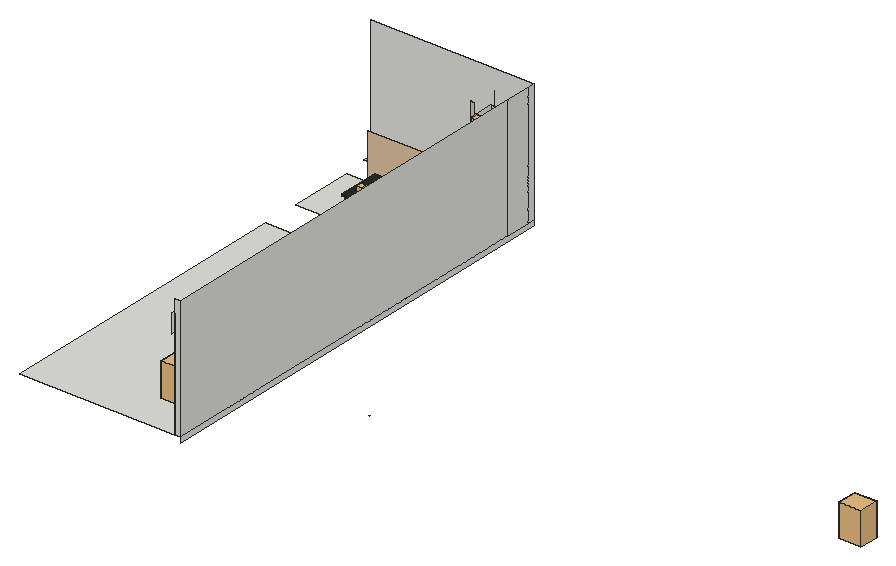
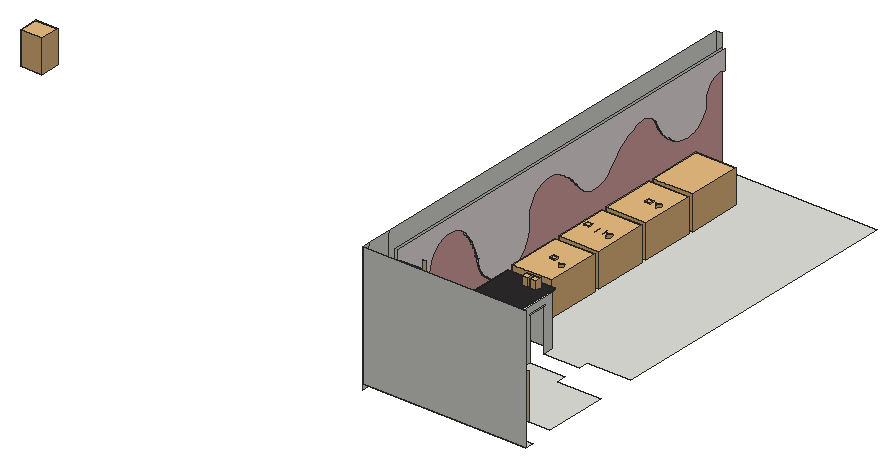
# SketchUp Ruby script. Lengths in inches.
U = 1.inch
M = Sketchup.active_model
def pt(a) = Geom::Point3d.new(a.map { |v| v * U })
def face(e, loops, mat)
  f = e.add_face(loops[0].map { |a| pt(a) })
  loops[1..].each { |l| e.add_face(l.map { |a| pt(a) }).erase! }
  f.material = f.back_material = mat if mat
  f
end
# faces: each face lists its corners as indices into pts; further lists are holes
def faces(e, pts, list, mat = nil) = list.each { |f| face(e, (f[0].is_a?(Array) ? f : [f]).map { |l| l.map { |i| pts[i] } }, mat) }
# xy, xz, yz: faces in a plane at the given z, y or x. An outline is a flat list of corners, or four numbers for a rectangle; further outlines are holes
def ring(l) = l.size == 4 ? [[l[0], l[1]], [l[2], l[1]], [l[2], l[3]], [l[0], l[3]]] : l.each_slice(2).to_a
def flat(e, list, mat, &to3) = list.each { |f| face(e, (f[0].is_a?(Array) ? f : [f]).map { |l| ring(l).map { |u, v| to3.(u, v) } }, mat) }
def xy(e, z, list, mat = nil) = flat(e, list, mat) { |x, y| [x, y, z] }
def xz(e, y, list, mat = nil) = flat(e, list, mat) { |x, z| [x, y, z] }
def yz(e, x, list, mat = nil) = flat(e, list, mat) { |y, z| [x, y, z] }
def lines(e, pts, list) = list.each { |a, b| e.add_line(pt(pts[a]), pt(pts[b])) }
# prism: a flat outline (further loops are holes) pulled along v
def prism(e, loops, v, mat = nil)
  f = face(e, loops, mat); d = Geom::Vector3d.new(v.map { |x| x * U })
  f.pushpull(f.normal.samedirection?(d) ? d.length : -d.length)
end
def box(e, o, s, mat = nil) = prism(e, [[o, [o[0] + s[0], o[1], o[2]], [o[0] + s[0], o[1] + s[1], o[2]], [o[0], o[1] + s[1], o[2]]]], [0, 0, s[2]], mat)
def at(x, y, z, deg = 0) = Geom::Transformation.translation(pt([x, y, z])) * Geom::Transformation.rotation(ORIGIN, Z_AXIS, deg.degrees)
def axes(o, x, y, z) = Geom::Transformation.new([*x, 0, *y, 0, *z, 0, *pt(o).to_a, 1])
def part(name) = M.definitions.add(name)
# library, detail: a bought-in or finely detailed component or shape, given as its bounding box
def library(name, o, s) = part(name).tap { |d| box(d.entities, o, s) }
def detail(e, o, s) = box(e.add_group.entities, o, s)
def put(e, d, t, mat = nil) = e.add_instance(d, t).tap { |i| i.material = mat if mat }
def group(e, t, mat = nil) = e.add_group.tap { |g| g.transformation = t; g.material = mat if mat }.entities
root = M.entities
M.materials.add("Generic").color = [224, 169, 169]
M.materials.add("Generic\#1").color = [44, 42, 42]
M.materials.add("Generic\#2").color = [246, 234, 234]
M.materials.add("Generic\#3").color = [224, 196, 161]
M.materials.add("Material__1").color = [51, 42, 44]
M.materials.add("Material__2").color = [97, 132, 37]
M.materials.add("[Color M00]").color = [255, 255, 255]
M.materials.add("[Mirror 02]").color = [230, 230, 230]
M.materials.add("[Translucent Glass Tinted]").color = [7, 201, 240]
M.materials["[Translucent Glass Tinted]"].alpha = 0.48
c1 = library("coffee+cup+lid",[0,0,0.03],[3.7,3.7,4.95])
c2 = library("\#1",[-138.85,-135.75,0],[277.7,270.97,9.64])
c3 = library("\#2",[-34.84,-73.35,-33.91],[69.68,146.26,68.31])
c4 = library("\#5",[-4127.85,-1300.75,-2324.72],[5349.84,4521.24,5423.31])
c5 = part("\#3")
put(c5.entities,c4,at(450.18,-1111.4375,0),"Material__2")
c6 = part("12")
put(c6.entities,c2,axes([-49.79,-36.9375,349.64],[0.59279,0,0],[0,0.59279,0],[0,0,0.59279]),"Material__1")
put(c6.entities,c3,axes([-39.24,-18.18,177.19],[1.20819,-2.09264,0],[0,0,2.41638],[2.09264,1.20819,0]))
put(c6.entities,c5,axes([-83.44,-46.04,442.44],[-0.03636,-0.03293,-0.01473],[-0.00083,-0.02391,0.05549],[0.02997,-0.02791,-0.01158]))
c7 = part("Group\#585")
xy(c7.entities,2.68,[[0,0,4.06,4.25]],"[Color M00]")
xz(c7.entities,0,[[0,0,4.06,2.68]],"[Color M00]")
xz(c7.entities,4.25,[[0,0,4.06,2.68]],"[Color M00]")
yz(c7.entities,0,[[0,0,4.25,2.68]],"[Color M00]")
yz(c7.entities,4.06,[[0,0,4.25,2.68]],"[Color M00]")
c8 = library("Tissue box",[0,0,0],[4.59,4,6.84])
c9 = library("Group\#665",[0,0,0],[25.17,25.17,22.5])
c10 = library("Group\#77",[0,0,0],[37.5,57.43,36.06])
c11 = library("Group\#78",[0,0,0],[37.5,57.43,36.06])
c12 = library("Group\#79",[0,0,0],[37.5,57.43,36.06])
c13 = library("Group\#80",[0,0,0],[37.5,57.43,36.06])
c14 = library("Group\#661",[0,0,0],[62.4,40.28,25.88])
xy(root,0,[[184.0625,0,190,453.375],[180.77,453.375,190,481.125],[153.2,476.9375,180.77,476.9375,180.77,481.125,190,481.125,190,490.125,9,490.125,9,481.125,153.2,481.125]])
xy(root,58.4375,[[97.8125,338.55,149.9375,340.55],[97.8125,340.55,99.75,382.3],[99.75,340.55,147.9375,382.3],[147.9375,340.55,149.9375,384.3],[97.8125,382.3,147.9375,384.3]])
xy(root,60.3125,[[97.8125,338.55,149.9375,384.3]],"Generic\#1")
xz(root,0,[[184.0625,0,190,135.25]])
xz(root,338.55,[[97.8125,58.4375,149.9375,60.3125]],"Generic\#1")
xz(root,340.55,[[99.75,0,147.9375,58.4375]])
xz(root,382.3,[[99.75,0,147.9375,58.4375]])
xz(root,384.3,[[97.8125,58.4375,149.9375,60.3125]])
xz(root,453.375,[[180.77,0,184.0625,0,184.0625,75.96,180.9375,75.96,180.9375,120,180.77,120],[184.0625,0,190,67.8125]])
xz(root,453.375,[[34.875,0,153.2,0,153.2,120,149.93,120,149.93,89.18,150.375,89.18,150.375,71.49,150.42,68.36,150.42,50.68,35.21,50.68,35.29,46.12]],"Generic\#3")
xz(root,476.9375,[[153.2,0,180.77,107.14]])
xz(root,490.125,[[9,0,190,135.25]])
yz(root,99.75,[[340.55,0,340.55,58.4375,382.3,58.4375,382.3,0,371.55,0,371.55,47.6875,372.8,47.6875,372.8,48.3125,350.05,48.3125,350.05,47.6875,351.3,47.6875,351.3,0],[350.05,47.6875,372.8,48.3125]])
yz(root,147.9375,[[340.55,0,382.3,58.4375]])
yz(root,149.9375,[[338.55,58.4375,384.3,60.3125]],"Generic\#1")
yz(root,150.42,[[453.375,50.68,476.6875,68.36]],"Generic\#3")
yz(root,150.79,[[453.375,45.99,467.1875,46.12]])
yz(root,153.2,[[453.375,0,476.9375,107.14]])
yz(root,180.77,[[453.375,0,476.9375,107.14]])
yz(root,180.9375,[[309.3,28.65,300.48,28.89,292.02,31.36,284.45,35.875,278.27,42.16,273.87,49.8,271.54,58.3,271.43,67.11,271.55,72.61,270.64,78.03,268.73,83.18,265.88,87.89,262.21,91.98,257.84,95.3125,252.92,97.77,247.63,99.26,242.16,99.73,236.6875,99.18,231.42,97.61,226.54,95.08,224.11,93.46,221.73,91.77,219.41,90.01,217.14,88.18,214.93,86.28,212.78,84.31,210.68,82.27,208.66,80.17,206.7,78.01,204.8,75.8,202.98,73.52,201.22,71.1875,198.44,67.94,195.19,65.17,191.55,62.95,187.6,61.31,183.45,60.32,179.1875,59.98,174.93,60.32,170.78,61.31,166.83,62.95,163.1875,65.17,159.9375,67.94,157.16,71.1875,154.72,74.36,152.1,77.39,149.34,80.28,146.41,83.01,143.35,85.58,140.15,87.99,136.83,90.22,133.39,92.26,129.85,94.12,126.21,95.79,122.48,97.25,118.6875,98.51,116.17,99.11,113.59,99.4,111,99.36,108.43,99.01,105.93,98.35,103.52,97.38,101.25,96.13,99.15,94.61,97.26,92.84,95.59,90.85,94.18,88.68,93.05,86.35,91.38,82.68,89.4375,79.15,87.23,75.77,84.78,72.57,82.09,69.57,79.1875,66.78,76.08,64.21,72.79,61.88,69.33,59.8125,65.72,58.01,61.99,56.48,58.16,55.24,54.1875,54.44,50.14,54.28,46.12,54.74,42.22,55.83,38.53,57.51,35.16,59.75,32.17,62.48,29.64,65.65,27.64,69.17,26.21,72.96,25.39,76.92,25.2,80.97,25.04,84,24.39,86.97,23.27,89.8,21.69,92.4,19.72,94.71,17.39,96.67,14.78,98.22,11.95,99.33,8.97,99.96,5.9375,100.09,2.92,99.73,0,98.88,0,120,453.375,120,453.375,75.96,452.625,70.25,450.42,64.92,446.91,60.36,442.34,56.85,437.02,54.65,431.3125,53.89,425.6,54.65,420.28,56.85,415.71,60.36,412.21,64.92,410,70.25,409.25,75.96,408.67,81.6875,406.96,87.1875,404.1875,92.23,400.46,96.625,395.93,100.18,390.79,102.77,385.23,104.27,379.48,104.64,373.77,103.84,368.34,101.93,363.4,98.97,359.15,95.08,356.78,92.31,354.54,89.43,352.42,86.46,350.45,83.4,348.6,80.25,346.9,77.02,345.35,73.73,343.94,70.36,342.6875,66.9375,341.58,63.46,340.64,59.9375,339.85,56.38,337.04,48.02,332.22,40.64,325.7,34.72,317.89,30.63]],"Generic\#2")
yz(root,184.0625,[[309.3,28.65,317.89,30.63,325.7,34.72,332.22,40.64,337.04,48.02,339.85,56.38,340.64,59.9375,341.58,63.46,342.6875,66.9375,343.94,70.36,345.35,73.73,346.9,77.02,348.6,80.25,350.45,83.4,352.42,86.46,354.54,89.43,356.78,92.31,359.15,95.08,363.4,98.97,368.34,101.93,373.77,103.84,379.48,104.64,385.23,104.27,390.79,102.77,395.93,100.18,400.46,96.625,404.1875,92.23,406.96,87.1875,408.67,81.6875,409.25,75.96,410,70.25,412.21,64.92,415.71,60.36,420.28,56.85,425.6,54.65,431.3125,53.89,437.02,54.65,442.34,56.85,446.91,60.36,450.42,64.92,452.625,70.25,453.375,75.96,453.375,120,0,120,0,98.88,2.92,99.73,5.9375,100.09,8.97,99.96,11.95,99.33,14.78,98.22,17.39,96.67,19.72,94.71,21.69,92.4,23.27,89.8,24.39,86.97,25.04,84,25.2,80.97,25.39,76.92,26.21,72.96,27.64,69.17,29.64,65.65,32.17,62.48,35.16,59.75,38.53,57.51,42.22,55.83,46.12,54.74,50.14,54.28,54.1875,54.44,58.16,55.24,61.99,56.48,65.72,58.01,69.33,59.8125,72.79,61.88,76.08,64.21,79.1875,66.78,82.09,69.57,84.78,72.57,87.23,75.77,89.4375,79.15,91.38,82.68,93.05,86.35,94.18,88.68,95.59,90.85,97.26,92.84,99.15,94.61,101.25,96.13,103.52,97.38,105.93,98.35,108.43,99.01,111,99.36,113.59,99.4,116.17,99.11,118.6875,98.51,122.48,97.25,126.21,95.79,129.85,94.12,133.39,92.26,136.83,90.22,140.15,87.99,143.35,85.58,146.41,83.01,149.34,80.28,152.1,77.39,154.72,74.36,157.16,71.1875,159.9375,67.94,163.1875,65.17,166.83,62.95,170.78,61.31,174.93,60.32,179.1875,59.98,183.45,60.32,187.6,61.31,191.55,62.95,195.19,65.17,198.44,67.94,201.22,71.1875,202.98,73.52,204.8,75.8,206.7,78.01,208.66,80.17,210.68,82.27,212.78,84.31,214.93,86.28,217.14,88.18,219.41,90.01,221.73,91.77,224.11,93.46,226.54,95.08,231.42,97.61,236.6875,99.18,242.16,99.73,247.63,99.26,252.92,97.77,257.84,95.3125,262.21,91.98,265.88,87.89,268.73,83.18,270.64,78.03,271.55,72.61,271.43,67.11,271.54,58.3,273.87,49.8,278.27,42.16,284.45,35.875,292.02,31.36,300.48,28.89]])
yz(root,184.0625,[[0,0,0,98.88,2.92,99.73,5.9375,100.09,8.97,99.96,11.95,99.33,14.78,98.22,17.39,96.67,19.72,94.71,21.69,92.4,23.27,89.8,24.39,86.97,25.04,84,25.2,80.97,25.39,76.92,26.21,72.96,27.64,69.17,29.64,65.65,32.17,62.48,35.16,59.75,38.53,57.51,42.22,55.83,46.12,54.74,50.14,54.28,54.1875,54.44,58.16,55.24,61.99,56.48,65.72,58.01,69.33,59.8125,72.79,61.88,76.08,64.21,79.1875,66.78,82.09,69.57,84.78,72.57,87.23,75.77,89.4375,79.15,91.38,82.68,93.05,86.35,94.18,88.68,95.59,90.85,97.26,92.84,99.15,94.61,101.25,96.13,103.52,97.38,105.93,98.35,108.43,99.01,111,99.36,113.59,99.4,116.17,99.11,118.6875,98.51,122.48,97.25,126.21,95.79,129.85,94.12,133.39,92.26,136.83,90.22,140.15,87.99,143.35,85.58,146.41,83.01,149.34,80.28,152.1,77.39,154.72,74.36,157.16,71.1875,159.9375,67.94,163.1875,65.17,166.83,62.95,170.78,61.31,174.93,60.32,179.1875,59.98,183.45,60.32,187.6,61.31,191.55,62.95,195.19,65.17,198.44,67.94,201.22,71.1875,202.98,73.52,204.8,75.8,206.7,78.01,208.66,80.17,210.68,82.27,212.78,84.31,214.93,86.28,217.14,88.18,219.41,90.01,221.73,91.77,224.11,93.46,226.54,95.08,231.42,97.61,236.6875,99.18,242.16,99.73,247.63,99.26,252.92,97.77,257.84,95.3125,262.21,91.98,265.88,87.89,268.73,83.18,270.64,78.03,271.55,72.61,271.43,67.11,271.54,58.3,273.87,49.8,278.27,42.16,284.45,35.875,292.02,31.36,300.48,28.89,309.3,28.65,317.89,30.63,325.7,34.72,332.22,40.64,337.04,48.02,339.85,56.38,340.64,59.9375,341.58,63.46,342.6875,66.9375,343.94,70.36,345.35,73.73,346.9,77.02,348.6,80.25,350.45,83.4,352.42,86.46,354.54,89.43,356.78,92.31,359.15,95.08,363.4,98.97,368.34,101.93,373.77,103.84,379.48,104.64,385.23,104.27,390.79,102.77,395.93,100.18,400.46,96.625,404.1875,92.23,406.96,87.1875,408.67,81.6875,409.25,75.96,410,70.25,412.21,64.92,415.71,60.36,420.28,56.85,425.6,54.65,431.3125,53.89,437.02,54.65,442.34,56.85,446.91,60.36,450.42,64.92,452.625,70.25,453.375,75.96,453.375,0]],"Generic")
yz(root,190,[[0,-6,490.125,0],[0,0,453.375,135.25],[453.375,0,481.125,135.25],[481.125,0,490.125,135.25]])
p = [[184.0625,309.3,28.65],[184.0625,300.48,28.89],[180.9375,300.48,28.89],[180.9375,309.3,28.65],[184.0625,317.89,30.63],[180.9375,317.89,30.63],
  [184.0625,292.02,31.36],[180.9375,292.02,31.36],[184.0625,325.7,34.72],[180.9375,325.7,34.72],[184.0625,284.45,35.875],[180.9375,284.45,35.875],
  [184.0625,332.22,40.64],[180.9375,332.22,40.64],[184.0625,278.27,42.16],[180.9375,278.27,42.16],[184.0625,337.04,48.02],[180.9375,337.04,48.02],
  [184.0625,273.87,49.8],[180.9375,273.87,49.8],[184.0625,339.85,56.38],[180.9375,339.85,56.38],[184.0625,271.54,58.3],[180.9375,271.54,58.3],
  [184.0625,431.3125,53.89],[184.0625,425.6,54.65],[180.9375,425.6,54.65],[180.9375,431.3125,53.89],[184.0625,437.02,54.65],[180.9375,437.02,54.65],
  [184.0625,50.14,54.28],[184.0625,46.12,54.74],[180.9375,46.12,54.74],[180.9375,50.14,54.28],[184.0625,54.1875,54.44],[180.9375,54.1875,54.44],
  [184.0625,58.16,55.24],[180.9375,58.16,55.24],[184.0625,420.28,56.85],[180.9375,420.28,56.85],[184.0625,442.34,56.85],[180.9375,442.34,56.85],
  [184.0625,42.22,55.83],[180.9375,42.22,55.83],[184.0625,61.99,56.48],[180.9375,61.99,56.48],[184.0625,38.53,57.51],[180.9375,38.53,57.51],
  [184.0625,340.64,59.9375],[180.9375,340.64,59.9375],[184.0625,65.72,58.01],[180.9375,65.72,58.01],[184.0625,415.71,60.36],[180.9375,415.71,60.36],
  [184.0625,446.91,60.36],[180.9375,446.91,60.36],[184.0625,35.16,59.75],[180.9375,35.16,59.75],[184.0625,69.33,59.8125],[180.9375,69.33,59.8125],
  [184.0625,271.43,67.11],[180.9375,271.43,67.11],[184.0625,32.17,62.48],[180.9375,32.17,62.48],[184.0625,72.79,61.88],[180.9375,72.79,61.88],
  [184.0625,341.58,63.46],[180.9375,341.58,63.46],[184.0625,179.1875,59.98],[184.0625,174.93,60.32],[180.9375,174.93,60.32],[180.9375,179.1875,59.98],
  [184.0625,183.45,60.32],[180.9375,183.45,60.32],[184.0625,170.78,61.31],[180.9375,170.78,61.31],[184.0625,187.6,61.31],[180.9375,187.6,61.31],
  [184.0625,412.21,64.92],[180.9375,412.21,64.92],[184.0625,450.42,64.92],[180.9375,450.42,64.92],[184.0625,166.83,62.95],[180.9375,166.83,62.95],
  [184.0625,191.55,62.95],[180.9375,191.55,62.95],[184.0625,76.08,64.21],[180.9375,76.08,64.21],[184.0625,29.64,65.65],[180.9375,29.64,65.65],
  [184.0625,163.1875,65.17],[180.9375,163.1875,65.17],[184.0625,195.19,65.17],[180.9375,195.19,65.17],[184.0625,342.6875,66.9375],[180.9375,342.6875,66.9375],
  [184.0625,79.1875,66.78],[180.9375,79.1875,66.78],[294.32,130.76,0],[295.32,130.76,0],[295.32,131.76,0],[150.79,467.1875,46.12],
  [150.42,467.1875,68.36],[180.77,481.125,120],[180.77,481.125,0],[153.2,481.125,120],[153.2,481.125,0]]
faces(root,p,[[0,1,2,3],[4,0,3,5],[1,6,7,2],[8,4,5,9],[6,10,11,7],[12,8,9,13],[10,14,15,11],[16,12,13,17],
  [14,18,19,15],[20,16,17,21],[18,22,23,19],[24,25,26,27],[28,24,27,29],[30,31,32,33],[34,30,33,35],[36,34,35,37],
  [25,38,39,26],[40,28,29,41],[31,42,43,32],[42,46,47,43],[38,52,53,39],[54,40,41,55],[46,56,57,47],[22,60,61,23],
  [56,62,63,57],[68,69,70,71],[72,68,71,73],[69,74,75,70],[76,72,73,77],[52,78,79,53],[80,54,55,81],[74,82,83,75],
  [84,76,77,85],[62,88,89,63],[82,90,91,83],[92,84,85,93]],"Generic\#2")
faces(root,p,[[44,36,37,45],[48,20,21,49],[50,44,45,51],[58,50,51,59],[64,58,59,65],[66,48,49,67],[86,64,65,87],[94,66,67,95],
  [96,86,87,97]])
lines(root,p,[[98,99],[99,100],[100,98],[101,102],[103,104],[105,106]])
g1 = group(root,at(12.375,0,0))
xy(g1,0,[[0,0,171.6875,0,171.6875,453.375,0,453.375,0,382.3,48.1875,382.3,48.1875,371.55,87.375,371.55,87.375,382.3,135.5625,382.3,135.5625,340.55,87.375,340.55,87.375,351.3,48.1875,351.3,48.1875,340.55,0,340.55]])
put(root,c1,axes([108.58,345.02,60.26],[1.82498,0,0],[0,1.82498,0],[0,0,1.82498]))
put(root,c1,axes([117.72,345.02,60.26],[1.82498,0,0],[0,1.82498,0],[0,0,1.82498]))
put(root,c6,axes([144.89,137.57,30],[0.01602,0,0],[0,0.01602,0],[0,0,0.01602]))
put(root,c6,axes([144.89,206.02,30],[0.01602,0,0],[0,0.01602,0],[0,0,0.01602]))
put(root,c6,axes([144.89,272.52,30],[0.01602,0,0],[0,0.01602,0],[0,0,0.01602]))
g2 = group(root,at(143.3,197.64,30))
xy(g2,0,[[3.57,1.44,4.14,1.51,4.66,1.71,5.12,2.05,5.47,2.49,5.7,3.01,5.78,3.57,5.72,4.14,5.51,4.66,5.17,5.12,4.73,5.47,4.21,5.7,3.65,5.78,3.09,5.72,2.56,5.51,2.11,5.17,1.75,4.73,1.53,4.21,1.44,3.65,1.51,3.09,1.71,2.56,2.05,2.11,2.49,1.75,3.01,1.53]],"[Mirror 02]")
xy(g2,2.03,[[[3.55,0,4.48,0.11,5.36,0.45,6.12,1.01,6.71,1.75,7.08,2.61,7.22,3.55,7.12,4.48,6.77,5.36,6.21,6.12,5.47,6.71,4.61,7.08,3.68,7.22,2.74,7.12,1.86,6.77,1.1,6.21,0.52,5.47,0.14,4.61,0,3.68,0.11,2.74,0.45,1.86,1.01,1.1,1.75,0.52,2.61,0.14],[3.55,0.17,2.66,0.31,1.84,0.67,1.14,1.22,0.6,1.95,0.28,2.78,0.17,3.67,0.31,4.56,0.67,5.38,1.22,6.08,1.95,6.62,2.78,6.95,3.67,7.05,4.56,6.91,5.38,6.56,6.08,6,6.62,5.28,6.95,4.44,7.05,3.55,6.91,2.66,6.56,1.84,6,1.14,5.28,0.6,4.44,0.28]]],"[Translucent Glass Tinted]")
p = [[2.61,0.14,2.03],[3.01,1.53,0],[3.57,1.44,0],[3.55,0,2.03],[4.14,1.51,0],[4.48,0.11,2.03],
  [1.75,0.52,2.03],[2.49,1.75,0],[4.66,1.71,0],[5.36,0.45,2.03],[1.01,1.1,2.03],[2.05,2.11,0],
  [5.12,2.05,0],[6.12,1.01,2.03],[5.47,2.49,0],[6.71,1.75,2.03],[0.45,1.86,2.03],[1.71,2.56,0],
  [5.7,3.01,0],[7.08,2.61,2.03],[0.11,2.74,2.03],[1.51,3.09,0],[5.78,3.57,0],[7.22,3.55,2.03],
  [0,3.68,2.03],[1.44,3.65,0],[5.72,4.14,0],[7.12,4.48,2.03],[1.53,4.21,0],[0.14,4.61,2.03],
  [5.51,4.66,0],[6.77,5.36,2.03],[1.75,4.73,0],[0.52,5.47,2.03],[2.11,5.17,0],[1.1,6.21,2.03],
  [5.17,5.12,0],[6.21,6.12,2.03],[4.73,5.47,0],[5.47,6.71,2.03],[2.56,5.51,0],[1.86,6.77,2.03],
  [3.09,5.72,0],[2.74,7.12,2.03],[4.21,5.7,0],[4.61,7.08,2.03],[3.65,5.78,0],[3.68,7.22,2.03]]
faces(g2,p,[[0,1,2,3],[3,2,4,5],[6,7,1,0],[5,4,8,9],[10,11,7,6],[9,8,12,13],[13,12,14,15],[16,17,11,10],
  [15,14,18,19],[20,21,17,16],[19,18,22,23],[24,25,21,20],[22,26,27,23],[28,25,24,29],[26,30,31,27],[32,28,29,33],
  [34,32,33,35],[30,36,37,31],[36,38,39,37],[40,34,35,41],[42,40,41,43],[38,44,45,39],[46,42,43,47],[44,46,47,45]],"[Translucent Glass Tinted]")
put(g2,c7,axes([1.18,1.99,1.13],[0.29618,0,0],[0,0.29618,0],[0,0,0.29618]))
put(g2,c7,axes([2.64,0.68,1.13],[0.29618,0,0],[0,0.29618,0],[0,0,0.29618]))
put(g2,c7,axes([3.69,3.57,0],[0.29618,0,0],[0,0.29618,0],[0,0,0.29618]))
put(g2,c7,axes([2.23,1.99,0],[0.29618,0,0],[0,0.29618,0],[0,0,0.29618]))
put(g2,c7,axes([3.99,3.57,1.13],[0.29618,0,0],[0,0.29618,0],[0,0,0.29618]))
put(g2,c7,axes([3.69,1.99,0],[0.29618,0,0],[0,0.29618,0],[0,0,0.29618]))
put(g2,c7,axes([1.18,3.57,1.13],[0.29618,0,0],[0,0.29618,0],[0,0,0.29618]))
put(g2,c7,axes([3.99,1.99,1.13],[0.29618,0,0],[0,0.29618,0],[0,0,0.29618]))
put(g2,c7,axes([2.64,3.57,1.13],[0.29618,0,0],[0,0.29618,0],[0,0,0.29618]))
put(g2,c7,axes([2.23,3.57,0],[0.29618,0,0],[0,0.29618,0],[0,0,0.29618]))
put(g2,c7,axes([2.64,1.99,1.13],[0.29618,0,0],[0,0.29618,0],[0,0,0.29618]))
put(root,c8,axes([152.6875,133.56,30],[1.16688,0,0],[0,1.16688,0],[0,0,1.16688]))
put(root,c9,axes([151.8,199.13,30.12],[0.3016,0,0],[0,0.3016,0],[0,0,0.3016]))
put(root,c10,axes([134.39,237.66,0],[1.17902,0,0],[0,1.0324,0],[0,0,1.0324]))
put(root,c11,axes([134.39,172.66,0],[1.17902,0,0],[0,1.0324,0],[0,0,1.0324]))
put(root,c12,axes([134.39,107.66,0],[1.17902,0,0],[0,1.0324,0],[0,0,1.0324]))
put(root,c13,axes([134.39,42.66,0],[1.17902,0,0],[0,1.0324,0],[0,0,1.0324]))
put(root,c8,axes([154.95,262.92,30],[1.16688,0,0],[0,1.16688,0],[0,0,1.16688]))
put(root,c14,axes([160.47,208.61,30.21],[0,-0.18,0],[0.18,0,0],[0,0,0.18]))
g3 = group(root,at(153.2,448.4375,0),"Generic\#3")
p = [[5.04,5.9375,54.21],[5.04,0,54.21]]
lines(g3,p,[[0,1]])
detail(g3,[0,0,0],[27.5625,7.75,107.14])
put(root,c8,axes([169,197.93,30],[1.16688,0,0],[0,1.16688,0],[0,0,1.16688]))
put(root,c8,axes([747.75,216.25,0],[5.28,0,0],[0,5.28,0],[0,0,5.28]))
